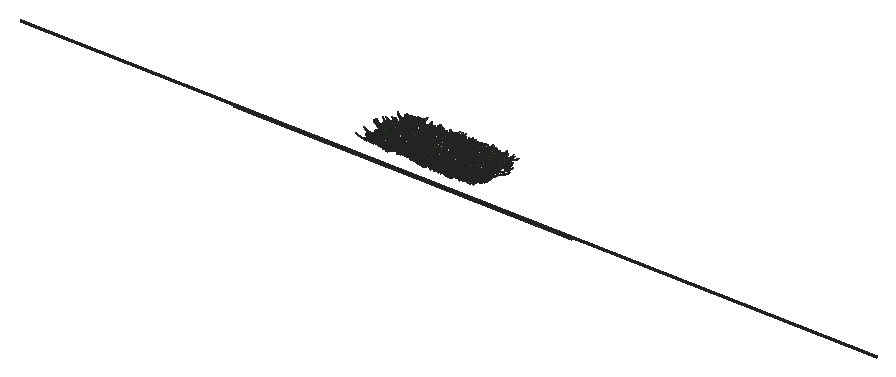
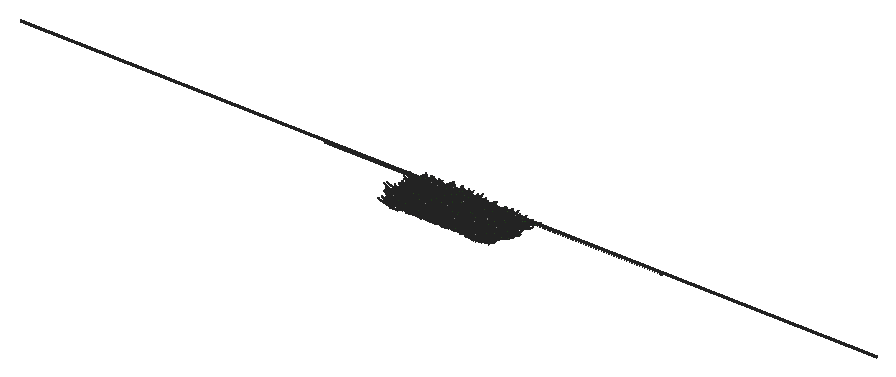
# SketchUp Ruby script. Lengths in inches.
U = 1.inch
M = Sketchup.active_model
def pt(a) = Geom::Point3d.new(a.map { |v| v * U })
def face(e, loops, mat)
  f = e.add_face(loops[0].map { |a| pt(a) })
  loops[1..].each { |l| e.add_face(l.map { |a| pt(a) }).erase! }
  f.material = f.back_material = mat if mat
  f
end
# faces: each face lists its corners as indices into pts; further lists are holes
def faces(e, pts, list, mat = nil) = list.each { |f| face(e, (f[0].is_a?(Array) ? f : [f]).map { |l| l.map { |i| pts[i] } }, mat) }
# xy, xz, yz: faces in a plane at the given z, y or x. An outline is a flat list of corners, or four numbers for a rectangle; further outlines are holes
def ring(l) = l.size == 4 ? [[l[0], l[1]], [l[2], l[1]], [l[2], l[3]], [l[0], l[3]]] : l.each_slice(2).to_a
def flat(e, list, mat, &to3) = list.each { |f| face(e, (f[0].is_a?(Array) ? f : [f]).map { |l| ring(l).map { |u, v| to3.(u, v) } }, mat) }
def xy(e, z, list, mat = nil) = flat(e, list, mat) { |x, y| [x, y, z] }
def xz(e, y, list, mat = nil) = flat(e, list, mat) { |x, z| [x, y, z] }
def yz(e, x, list, mat = nil) = flat(e, list, mat) { |y, z| [x, y, z] }
def lines(e, pts, list) = list.each { |a, b| e.add_line(pt(pts[a]), pt(pts[b])) }
# prism: a flat outline (further loops are holes) pulled along v
def prism(e, loops, v, mat = nil)
  f = face(e, loops, mat); d = Geom::Vector3d.new(v.map { |x| x * U })
  f.pushpull(f.normal.samedirection?(d) ? d.length : -d.length)
end
def box(e, o, s, mat = nil) = prism(e, [[o, [o[0] + s[0], o[1], o[2]], [o[0] + s[0], o[1] + s[1], o[2]], [o[0], o[1] + s[1], o[2]]]], [0, 0, s[2]], mat)
def at(x, y, z, deg = 0) = Geom::Transformation.translation(pt([x, y, z])) * Geom::Transformation.rotation(ORIGIN, Z_AXIS, deg.degrees)
def axes(o, x, y, z) = Geom::Transformation.new([*x, 0, *y, 0, *z, 0, *pt(o).to_a, 1])
def part(name) = M.definitions.add(name)
# library, detail: a bought-in or finely detailed component or shape, given as its bounding box
def library(name, o, s) = part(name).tap { |d| box(d.entities, o, s) }
def detail(e, o, s) = box(e.add_group.entities, o, s)
def put(e, d, t, mat = nil) = e.add_instance(d, t).tap { |i| i.material = mat if mat }
def group(e, t, mat = nil) = e.add_group.tap { |g| g.transformation = t; g.material = mat if mat }.entities
root = M.entities
M.materials.add("Material82").color = [68, 110, 58]
M.materials.add("Material83").color = [48, 90, 38]
M.materials.add("Material84").color = [68, 110, 48]
M.materials.add("Material85").color = [48, 90, 48]
M.materials.add("Material86").color = [58, 110, 58]
M.materials.add("Material87").color = [58, 90, 38]
M.materials.add("Material88").color = [68, 100, 58]
M.materials.add("Material89").color = [48, 100, 38]
c1 = part("grass00")
p = [[-0.6875,0.15,0],[-0.56,0.08,5.52],[-0.04,0.03,2.76],[0.48,-0.02,0],[0.35,-0.02,5.52],[-0.1,-0.14,5.52],
  [-0.12,0.65,8.37],[-0.42,0.65,8.37]]
faces(c1.entities,p,[[0,1,2,3],[3,2,4],[1,5,2],[5,4,2],[1,6,5],[4,5,6],[7,6,1]])
c2 = part("Group16\#1")
put(c2.entities,c1,axes([1.44,-0.61,-0.01],[0.05352,0.12609,0],[-0.10704,0.04543,0.07239],[0.06664,-0.02828,0.11628]),"Material85")
put(c2.entities,c1,axes([0.76,-0.15,-0.01],[0.04676,0.24062,0],[-0.23162,0.04501,0.06642],[0.0652,-0.01267,0.23595]),"Material82")
put(c2.entities,c1,axes([0.79,0.01,-0.01],[-0.00606,0.34651,0],[-0.34381,-0.00602,0.0432],[0.04319,0.00076,0.34386]))
put(c2.entities,c1,axes([1,0.23,-0.01],[-0.07192,0.31144,0],[-0.28722,-0.06632,0.1236],[0.12043,0.02781,0.29478]),"Material84")
put(c2.entities,c1,axes([1.66,0.77,-0.01],[-0.13828,0.29651,0],[-0.21551,-0.1005,0.22471],[0.20365,0.09498,0.23779]),"Material89")
put(c2.entities,c1,axes([0.6875,0.52,-0.01],[-0.18126,0.24051,0],[-0.22746,-0.17142,0.09788],[0.07817,0.05891,0.28481]),"Material84")
put(c2.entities,c1,axes([0.68,0.78,-0.01],[-0.215,0.18688,0],[-0.12385,-0.14248,0.21334],[0.13995,0.16101,0.18878]),"Material82")
put(c2.entities,c1,axes([0.56,1,-0.01],[-0.13756,0.07624,0],[-0.06159,-0.11112,0.0927],[0.04494,0.08108,0.12705]),"Material84")
put(c2.entities,c1,axes([0.2,0.64,-0.01],[-0.23729,0.07254,0],[-0.05711,-0.18681,0.153],[0.04473,0.14632,0.19535]),"Material89")
put(c2.entities,c1,axes([0.0625,0.72,-0.01],[-0.28874,0.02525,0],[-0.02179,-0.24916,0.14647],[0.01276,0.14591,0.25012]),"Material82")
put(c2.entities,c1,axes([-0.08,0.62,-0.01],[-0.34089,-0.04187,0],[0.03255,-0.26504,0.216],[-0.02633,0.21439,0.26703]),"Material89")
put(c2.entities,c1,axes([-0.34,0.98,-0.01],[-0.14314,-0.0493,0],[0.04397,-0.12769,0.06843],[-0.02228,0.0647,0.13505]),"Material89")
put(c2.entities,c1,axes([-0.87,1.45,-0.01],[-0.23488,-0.14114,0],[0.13761,-0.22901,0.06087],[-0.03135,0.05217,0.26717]))
put(c2.entities,c1,axes([-0.72,0.77,-0.01],[-0.14208,-0.13251,0],[0.07209,-0.0773,0.16301],[-0.11118,0.11922,0.1057]),"Material89")
put(c2.entities,c1,axes([-0.62,0.43,-0.01],[-0.14845,-0.21203,0],[0.18654,-0.13061,0.12304],[-0.10079,0.07057,0.22772]),"Material82")
put(c2.entities,c1,axes([-0.68,0.29,-0.01],[-0.13639,-0.32136,0],[0.31723,-0.13464,0.05579],[-0.05136,0.0218,0.34462]),"Material83")
put(c2.entities,c1,axes([-0.64,0.125,-0.01],[-0.0458,-0.23569,0],[0.22124,-0.043,0.08276],[-0.08124,0.01579,0.22538]),"Material86")
put(c2.entities,c1,axes([-1.6,-0.03,-0.01],[0.00576,-0.32897,0],[0.27526,0.00482,0.18018],[-0.18015,-0.00315,0.2753]),"Material84")
put(c2.entities,c1,axes([-1.36,-0.31,-0.01],[0.05718,-0.24765,0],[0.18172,0.04196,0.17267],[-0.16825,-0.03885,0.1865]),"Material89")
put(c2.entities,c1,axes([-1.54,-0.72,-0.01],[0.06537,-0.14017,0],[0.13555,0.06321,0.03939],[-0.0357,-0.01665,0.14956]))
put(c2.entities,c1,axes([-1.19,-0.9,-0.01],[0.09597,-0.12735,0],[0.11214,0.08451,0.07557],[-0.06035,-0.04548,0.14042]),"Material88")
put(c2.entities,c1,axes([-0.47,-0.54,-0.01],[0.11588,-0.10072,0],[0.0618,0.0711,0.12124],[-0.07953,-0.0915,0.0942]))
put(c2.entities,c1,axes([-0.47,-0.84,-0.01],[0.11927,-0.0661,0],[0.06603,0.11913,0.00646],[-0.00313,-0.00565,0.13621]),"Material84")
put(c2.entities,c1,axes([-0.38,-1.24,-0.01],[0.28037,-0.08571,0],[0.0618,0.20215,0.20315],[-0.05939,-0.19428,0.21139]),"Material88")
put(c2.entities,c1,axes([-0.06,-0.66,-0.01],[0.22719,-0.01987,0],[0.01247,0.14255,0.17758],[-0.01547,-0.17691,0.1431]),"Material87")
put(c2.entities,c1,axes([0.11,-0.89,-0.01],[0.14882,0.01828,0],[-0.01058,0.08611,0.12229],[0.01491,-0.12138,0.08676]),"Material85")
put(c2.entities,c1,axes([0.25,-0.72,-0.01],[0.20481,0.07053,0],[-0.06206,0.18022,0.10291],[0.03351,-0.0973,0.1906]),"Material85")
put(c2.entities,c1,axes([0.85,-1.42,-0.01],[0.16481,0.09904,0],[-0.09472,0.15762,0.05616],[0.02893,-0.04814,0.18389]),"Material84")
put(c2.entities,c1,axes([1.01,-1.09,-0.01],[0.21858,0.20385,0],[-0.17495,0.1876,0.15339],[0.10462,-0.11218,0.25652]),"Material89")
put(c2.entities,c1,axes([1.01,-0.71,-0.01],[0.08733,0.12473,0],[-0.06445,0.04512,0.13037],[0.1068,-0.07477,0.07867]),"Material85")
c3 = part("Group15\#1")
put(c3.entities,c2,at(0,0,0))
c4 = part("3darcstudiotree_grass00\#1")
put(c4.entities,c3,at(0,0,0))
xz(root,273.41,[[626.68,-39.125,848.97,-38.61],[486.41,-38.1875,1048.66,-37.86],[486.41,-37.86,1048.66,-37.24]])
put(root,c4,axes([755.25,281.3125,-34.17],[3.22982,-1.36398,0],[2.52221,0.92889,-0.01281],[0.05669,0.02088,1.56626]))
put(root,c4,axes([763.375,281.07,-34.17],[0.45304,1.69594,0],[-3.37186,0.14009,-0.01763],[-0.11097,0.00461,1.60818]))
put(root,c4,axes([752.73,281.26,-34.17],[-2.98133,1.10226,0],[-2.6348,-1.10837,-0.04557],[-0.21161,-0.08902,1.96028]))
put(root,c4,axes([745.06,281.49,-34.17],[0.75696,1.65896,0],[-4.64105,0.32936,-0.03105],[-0.12997,0.00922,1.50318]))
put(root,c4,axes([773.35,281.36,-34.17],[-1.86859,1.14232,0],[-3.14905,-0.80116,-0.00439],[-0.02189,-0.00557,1.66469]))
put(root,c4,axes([719.16,282.96,-34.17],[3.31562,-0.63662,0],[1.81859,1.47309,-0.02466],[0.05194,0.04207,1.49812]))
put(root,c4,axes([769.54,282.6,-34.17],[2.60331,1.05125,0],[-2.58261,0.9947,-0.01838],[-0.08057,0.03103,1.65818]))
put(root,c4,axes([734.7,282.9375,-34.17],[4.09444,0.12503,0],[-0.31641,1.61154,-0.0417],[-0.02006,0.10219,1.91485]))
put(root,c4,axes([755.98,283.15,-34.17],[3.14565,-0.76847,0],[1.85222,1.17921,-0.00486],[0.01386,0.00882,1.42853]))
put(root,c4,axes([738.35,282.67,-34.17],[-0.14266,1.36173,0],[-4.10184,-0.06683,-0.00296],[-0.01424,-0.00023,1.47961]))
put(root,c4,axes([722.52,282.6,-34.17],[-3.65106,0.9561,0],[-2.55118,-1.5152,-0.05111],[-0.12576,-0.07469,1.53759]))
put(root,c4,axes([750.39,282.95,-34.17],[-3.45178,0.2701,0],[-0.90786,-1.80446,-0.05548],[-0.0508,-0.10098,1.6451]))
put(root,c4,axes([727.26,283.58,-34.17],[3.35024,-0.43777,0],[1.10858,1.31952,-0.03222],[0.06859,0.08164,1.78787]))
put(root,c4,axes([713.76,283.2,-34.17],[-4.08016,-0.15242,0],[0.34321,-1.42893,-0.02721],[0.0124,-0.05162,1.31849]))
put(root,c4,axes([772.58,283.29,-34.17],[-0.10583,1.54224,0],[-3.7996,-0.04055,-0.00627],[-0.03571,-0.00038,1.62459]))
put(root,c4,axes([743.97,283.65,-34.17],[-2.56709,-0.87628,0],[2.75862,-1.25691,-0.00422],[0.01164,-0.0053,1.33295]))
put(root,c4,axes([762.34,283.9,-34.17],[2.94971,1.39882,0],[-3.26889,1.07209,-0.02991],[-0.14108,0.04627,1.95467]))
put(root,c4,axes([739.51,284.71,-34.17],[3.68364,0.44666,0],[-1.28613,1.64968,-0.02064],[-0.02718,0.03487,1.46981]))
put(root,c4,axes([756.35,285.1,-34.17],[1.53079,-1.5017,0],[4.19952,0.6658,-0.01772],[0.08663,0.01374,1.7874]))
put(root,c4,axes([717.34,284.68,-34.17],[-0.8053,1.43922,0],[-4.1788,-0.36366,-0.05256],[-0.20936,-0.01822,1.30827]))
put(root,c4,axes([752.53,285.36,-34.17],[1.13972,-1.41461,0],[4.50389,0.56436,-0.03698],[0.18209,0.02282,1.82987]))
put(root,c4,axes([734.63,285.26,-34.17],[3.61655,0.77067,0],[-2.16585,1.58076,-0.05913],[-0.11484,0.08382,1.39517]))
put(root,c4,axes([745.85,285.29,-34.17],[-1.56362,-1.21345,0],[3.6466,-0.73082,-0.00876],[0.03709,-0.00743,1.45672]))
put(root,c4,axes([774.84,285.4,-34.17],[-3.61232,0.8121,0],[-2.24589,-1.55373,-0.01918],[-0.05035,-0.03483,1.80194]))
put(root,c4,axes([766.03,286.01,-34.17],[3.57437,0.42668,0],[-1.04232,1.35805,-0.0422],[-0.08519,0.111,1.87907]))
put(root,c4,axes([727.7,286.11,-34.17],[2.52987,0.96809,0],[-2.35442,0.95693,-0.00683],[-0.03278,0.01332,1.74693]))
put(root,c4,axes([724.6875,285.88,-34.17],[0.40934,1.39565,0],[-3.638,0.16595,-0.04522],[-0.26335,0.01201,1.60941]))
put(root,c4,axes([764.01,285.87,-34.17],[-3.36311,0.85521,0],[-1.93534,-1.1837,-0.01497],[-0.0443,-0.0271,1.4615]))
put(root,c4,axes([713.21,286.76,-34.17],[0.83554,-1.66698,0],[4.46376,0.34798,-0.04547],[0.22573,0.0176,1.72572]))
put(root,c4,axes([768.86,286.72,-34.17],[-0.65586,-1.46962,0],[4.60144,-0.31938,-0.05842],[0.32577,-0.02261,1.98292]))
put(root,c4,axes([727.76,286.96,-34.17],[0.10079,1.33733,0],[-4.05045,0.04748,-0.05613],[-0.28184,0.0033,1.5259]))
put(root,c4,axes([773.53,287.11,-34.17],[-0.80891,1.58211,0],[-4.50454,-0.3582,-0.03197],[-0.1625,-0.01292,1.78572]))
put(root,c4,axes([762.92,287.18,-34.17],[-2.18902,1.07825,0],[-2.9207,-0.92221,-0.02462],[-0.13408,-0.04234,1.95656]))
put(root,c4,axes([721.68,287.61,-34.17],[-2.79747,-0.82267,0],[2.4,-1.26929,-0.00029],[0.00098,-0.00052,1.69542]))
put(root,c4,axes([746.86,287.51,-34.17],[0.20899,1.64265,0],[-4.27343,0.08456,-0.03261],[-0.1888,0.00374,1.85888]))
put(root,c4,axes([735.6875,287.79,-34.17],[-3.83423,-0.51133,0],[1.38691,-1.61748,-0.06149],[0.1095,-0.1277,1.80385]))
put(root,c4,axes([758.12,288.25,-34.17],[0.38628,-1.42854,0],[3.50239,0.14729,-0.04937],[0.32013,0.01346,1.72169]))
put(root,c4,axes([718.66,287.69,-34.17],[-1.21632,1.56365,0],[-3.36368,-0.40694,-0.03727],[-0.21338,-0.02582,1.57911]))
put(root,c4,axes([741.22,287.77,-34.17],[-2.10873,0.99525,0],[-2.92476,-0.96381,-0.03387],[-0.14037,-0.04626,1.54303]))
put(root,c4,axes([733.14,289.03,-34.17],[4.32757,-0.42653,0],[1.12297,1.77206,-0.03338],[0.0321,0.05066,1.37691]))
put(root,c4,axes([753,288.3,-34.17],[-3.3677,0.38425,0],[-1.22656,-1.67195,-0.00573],[-0.0077,-0.0105,1.59925]))
put(root,c4,axes([750.55,289.42,-34.17],[4.24203,-0.02956,0],[0.08072,1.80172,-0.02875],[0.00231,0.05162,1.55972]))
put(root,c4,axes([730.76,289.23,-34.17],[-2.64283,-1.13535,0],[3.48014,-1.25993,-0.02326],[0.08818,-0.03192,1.82249]))
put(root,c4,axes([768.4,289.62,-34.17],[1.16933,-1.48396,0],[3.883,0.47588,-0.02169],[0.1048,0.01284,1.54236]))
put(root,c4,axes([755.74,289.61,-34.17],[3.86384,0.07818,0],[-0.23972,1.84255,-0.05168],[-0.01275,0.09801,1.68853]))
put(root,c4,axes([741.0625,289.94,-34.17],[3.33633,-0.58263,0],[1.85643,1.65335,-0.04981],[0.10311,0.09183,1.75709]))
put(root,c4,axes([718.1875,290.5,-34.17],[2.313,-1.43442,0],[2.99954,0.75225,-0.04064],[0.1888,0.04735,1.46692]))
put(root,c4,axes([773.14,290.52,-34.17],[0.21445,-1.64927,0],[3.6182,0.07317,-0.01161],[0.06174,0.00125,1.44612]))
put(root,c4,axes([744.34,290.38,-34.17],[2.09092,1.38555,0],[-3.43654,0.80658,-0.00188],[-0.01015,0.00238,1.87843]))
put(root,c4,axes([763.36,290.52,-34.17],[-2.42754,-1.16571,0],[2.71881,-0.88058,-0.021],[0.08634,-0.02796,1.40308]))
put(root,c4,axes([725.09,290.24,-34.17],[-2.97215,1.15542,0],[-3.15373,-1.26173,-0.01243],[-0.04576,-0.01831,1.76595]))
put(root,c4,axes([764.41,291.39,-34.17],[3.8213,1.10557,0],[-2.37941,1.27911,-0.00415],[-0.01079,0.0058,1.32509]))
put(root,c4,axes([717.7,291.5,-34.17],[3.43029,0.99275,0],[-1.97308,1.06035,-0.01519],[-0.04853,0.02608,1.34969]))
put(root,c4,axes([772.67,291.5,-34.17],[-3.1974,-0.52057,0],[1.31873,-1.25975,-0.01181],[0.03016,-0.02882,1.73426]))
put(root,c4,axes([751.76,291.51,-34.17],[-3.96689,-0.26306,0],[0.64548,-1.51387,-0.0114],[0.01279,-0.03,1.97478]))
put(root,c4,axes([744.57,292.32,-34.17],[3.4734,-0.75241,0],[2.06047,1.47936,-0.02691],[0.07219,0.05183,1.78778]))
put(root,c4,axes([730.22,292.4375,-34.17],[1.26532,-1.44178,0],[3.12553,0.42661,-0.00044],[0.00223,0.0003,1.32507]))
put(root,c4,axes([721.66,292.03,-34.17],[2.61816,1.29298,0],[-2.60516,0.82044,-0.01421],[-0.06264,0.01973,1.40932]))
put(root,c4,axes([738.7,292.6,-34.17],[2.17735,-1.14497,0],[3.55677,1.05197,-0.03529],[0.11494,0.03399,1.35654]))
put(root,c4,axes([736.05,291.86,-34.17],[-3.45507,0.18922,0],[-0.60525,-1.7188,-0.02154],[-0.01288,-0.03658,1.4342]))
put(root,c4,axes([758.55,291.99,-34.17],[0.41177,1.61489,0],[-3.5087,0.13914,-0.04963],[-0.27633,0.01096,1.47912]))
put(root,c4,axes([768.19,292.23,-34.17],[-3.24054,-0.28468,0],[0.77392,-1.37016,-0.02543],[0.03342,-0.05916,1.61262]))
put(root,c4,axes([729.84,293.65,-34.17],[3.40614,0.32781,0],[-0.81542,1.31776,-0.01459],[-0.02356,0.03807,1.75568]))
put(root,c4,axes([774.73,293.92,-34.17],[4.64374,0.18316,0],[-0.43015,1.69615,-0.02551],[-0.01161,0.04577,1.48132]))
put(root,c4,axes([741.5,293.4,-34.17],[-3.50392,-0.27669,0],[0.88512,-1.7433,-0.02406],[0.02146,-0.04227,1.53532]))
put(root,c4,axes([735.4375,293.52,-34.17],[1.33968,1.52005,0],[-3.16755,0.43419,-0.01128],[-0.07711,0.01057,1.81963]))
put(root,c4,axes([766.4,294.16,-34.17],[1.53865,-1.45346,0],[4.25105,0.69992,-0.03949],[0.18935,0.03118,1.7941]))
put(root,c4,axes([721.62,294,-34.17],[-3.43052,-0.93956,0],[2.00829,-1.14045,-0.00375],[0.01479,-0.0084,1.82358]))
put(root,c4,axes([749.93,294.53,-34.17],[-0.8562,-1.46222,0],[3.2715,-0.29793,-0.0292],[0.1741,-0.01586,1.53984]))
put(root,c4,axes([756.88,294.38,-34.17],[-3.12873,-1.31633,0],[2.88309,-1.0658,-0.03051],[0.12402,-0.04585,1.65027]))
put(root,c4,axes([716.5,294.17,-34.17],[1.08587,1.67228,0],[-4.264,0.43062,-0.00469],[-0.02209,0.00223,1.60422]))
put(root,c4,axes([713.79,294.57,-34.17],[-2.42435,1.35441,0],[-3.23148,-0.89962,-0.04566],[-0.20763,-0.0578,1.65042]))
put(root,c4,axes([746.87,294.8,-34.17],[-2.97303,0.61552,0],[-2.04085,-1.53313,-0.02543],[-0.06857,-0.05151,1.9093]))
put(root,c4,axes([729.625,295.45,-34.17],[0.04452,-1.40138,0],[3.5701,0.01764,-0.00992],[0.04898,0.00024,1.32167]))
put(root,c4,axes([763.46,294.86,-34.17],[-4.30499,0.20084,0],[-0.50439,-1.68151,-0.02284],[-0.01208,-0.04026,1.44864]))
put(root,c4,axes([753.09,295.68,-34.17],[-2.49551,-1.26471,0],[2.8619,-0.87828,-0.01663],[0.09126,-0.02801,1.89037]))
put(root,c4,axes([733.8125,296,-34.17],[3.17214,0.39156,0],[-1.05658,1.33127,-0.01935],[-0.04192,0.05282,1.92273]))
put(root,c4,axes([712.15,296.01,-34.17],[3.52761,0.55067,0],[-1.26989,1.26523,-0.04887],[-0.1287,0.12823,1.85053]))
put(root,c4,axes([720.16,296.8,-34.17],[3.22727,-0.96219,0],[2.40393,1.25403,-0.04167],[0.15655,0.08166,1.86151]))
put(root,c4,axes([765.95,296.79,-34.17],[1.36885,-1.43158,0],[3.98655,0.59286,-0.04892],[0.27754,0.04127,1.93615]))
put(root,c4,axes([761.17,296.19,-34.17],[-3.9685,0.8355,0],[-2.02289,-1.49439,-0.03463],[-0.09424,-0.06962,1.86049]))
put(root,c4,axes([725.1875,296.36,-34.17],[1.39622,1.62786,0],[-3.6301,0.48424,-0.04556],[-0.23124,0.03085,1.53888]))
put(root,c4,axes([739.57,296.34,-34.17],[-4.01589,0.275,0],[-0.74615,-1.69466,-0.05401],[-0.03733,-0.08478,1.3206]))
put(root,c4,axes([773.73,296.38,-34.17],[-3.10318,1.24143,0],[-2.60712,-1.01358,-0.05097],[-0.2393,-0.09303,1.80901]))
put(root,c4,axes([755.57,296.39,-34.17],[0.17144,1.84869,0],[-4.60552,0.06643,-0.0182],[-0.07619,0.0011,1.44668]))
put(root,c4,axes([746.52,296.81,-34.17],[2.02269,1.40625,0],[-2.88305,0.64496,-0.03898],[-0.27125,0.06068,1.98748]))
put(root,c4,axes([717.3,297.63,-34.17],[0.48715,-1.38403,0],[3.63737,0.19912,-0.0013],[0.00869,0.00048,1.85519]))
put(root,c4,axes([774.21,297.67,-34.17],[4.4529,0.04613,0],[-0.09862,1.48061,-0.04419],[-0.00818,0.12282,1.98467]))
put(root,c4,axes([763.3,297.87,-34.17],[-1.73285,-1.40976,0],[3.20349,-0.61242,-0.03263],[0.20579,-0.03934,1.87]))
put(root,c4,axes([741.37,297.76,-34.17],[0.25957,1.50579,0],[-3.94932,0.10588,-0.02807],[-0.1244,0.00334,1.3177]))
put(root,c4,axes([729.98,298.47,-34.17],[3.60093,0.62069,0],[-1.54425,1.39338,-0.01451],[-0.03218,0.02903,1.59989]))
put(root,c4,axes([769.54,298.41,-34.17],[-3.57377,-0.68668,0],[1.88387,-1.52489,-0.02869],[0.074,-0.0599,1.89824]))
put(root,c4,axes([722.57,298.84,-34.17],[4.25337,0.6683,0],[-1.56461,1.54873,-0.01606],[-0.02903,0.02874,1.54782]))
put(root,c4,axes([743.87,298.39,-34.17],[-2.10864,1.34219,0],[-3.56504,-0.87109,-0.01218],[-0.05259,-0.01285,1.59607]))
put(root,c4,axes([732.89,298.36,-34.17],[-2.73949,1.39402,0],[-3.69271,-1.12865,-0.03455],[-0.12332,-0.03769,1.58129]))
put(root,c4,axes([714.03,298.57,-34.17],[-4.29343,-0.7683,0],[1.85419,-1.61153,-0.00153],[0.00342,-0.00297,1.82565]))
put(root,c4,axes([750.54,299.13,-34.17],[-0.26486,1.49696,0],[-3.89065,-0.10706,-0.02357],[-0.1242,-0.00342,1.54387]))
put(root,c4,axes([718.5,299.89,-34.17],[2.27709,-1.12887,0],[2.96357,0.92974,-0.01848],[0.07518,0.02359,1.47553]))
put(root,c4,axes([757.24,299.24,-34.17],[-3.19374,0.7238,0],[-2.32014,-1.59223,-0.04948],[-0.1132,-0.07768,1.60238]))
put(root,c4,axes([755.24,300.34,-34.17],[4.72899,0.01401,0],[-0.03317,1.74196,-0.012],[-0.00046,0.02441,1.70791]))
put(root,c4,axes([733.2,300.48,-34.17],[-2.29669,-1.11112,0],[2.95834,-0.95105,-0.00371],[0.01505,-0.00484,1.4993]))
put(root,c4,axes([746.09,300.5,-34.17],[-3.17921,-1.35137,0],[3.1644,-1.15784,-0.01209],[0.04457,-0.01631,1.62724]))
put(root,c4,axes([772.52,300.76,-34.17],[-0.51556,-1.46046,0],[3.95081,-0.21691,-0.04493],[0.28513,-0.01565,1.91565]))
put(root,c4,axes([768.24,300.875,-34.17],[-1.16799,-1.2811,0],[3.57696,-0.50721,-0.0171],[0.1013,-0.01436,1.79343]))
put(root,c4,axes([763.83,300.54,-34.17],[0.87217,1.79185,0],[-4.36686,0.33058,-0.02457],[-0.1156,0.00875,1.59681]))
put(root,c4,axes([714.07,301.35,-34.17],[0.26653,-1.73376,0],[4.03869,0.09656,-0.02606],[0.1443,0.00345,1.68211]))
put(root,c4,axes([750.1875,301.02,-34.17],[-4.0045,-0.70324,0],[1.53901,-1.36302,-0.04343],[0.08424,-0.0746,1.35201]))
put(root,c4,axes([731.07,301.04,-34.17],[-0.93158,1.57452,0],[-3.64716,-0.33561,-0.02125],[-0.09909,-0.00912,1.34411]))
put(root,c4,axes([739.02,301.15,-34.17],[-1.92395,1.11114,0],[-2.73961,-0.73778,-0.01899],[-0.11099,-0.02989,1.75992]))
put(root,c4,axes([725.69,302.05,-34.17],[4.28281,-0.63976,0],[1.42181,1.48036,-0.01068],[0.01649,0.01717,1.31138]))
put(root,c4,axes([721.77,301.36,-34.17],[-3.74102,0.70585,0],[-1.92999,-1.5909,-0.05113],[-0.08819,-0.0727,1.33965]))
put(root,c4,axes([768.04,302.07,-34.17],[4.39904,-0.03006,0],[0.06093,1.38656,-0.04649],[0.00481,0.10943,1.57333]))
put(root,c4,axes([749.66,302.36,-34.17],[2.12424,-1.58648,0],[2.98317,0.62124,-0.03491],[0.20173,0.04201,1.65255]))
put(root,c4,axes([741.92,302.7,-34.17],[2.84805,-1.35819,0],[2.78081,0.90692,-0.04304],[0.21584,0.07039,1.76026]))
put(root,c4,axes([745.42,302.4,-34.17],[-1.97289,1.32597,0],[-3.97358,-0.91953,-0.01374],[-0.05147,-0.01191,1.50009]))
put(root,c4,axes([730.74,302.52,-34.17],[-4.13794,-0.2249,0],[0.58111,-1.66288,-0.00876],[0.00496,-0.01418,1.32289]))
put(root,c4,axes([755.37,302.74,-34.17],[1.47307,1.52241,0],[-3.55442,0.5349,-0.03212],[-0.18221,0.02742,1.73128]))
put(root,c4,axes([716.82,302.92,-34.17],[-4.03021,-0.53258,0],[1.1352,-1.33605,-0.02118],[0.04192,-0.04934,1.66873]))
put(root,c4,axes([771.67,303.0625,-34.17],[-4.17671,-0.8199,0],[2.05439,-1.62767,-0.0574],[0.10467,-0.08292,1.41402]))
put(root,c4,axes([760.75,303.1,-34.17],[-1.70053,1.52985,0],[-3.13018,-0.54115,-0.01229],[-0.08699,-0.01504,1.9803]))
put(root,c4,axes([736,303.53,-34.17],[-0.83712,1.35251,0],[-3.5635,-0.34303,-0.03757],[-0.17469,-0.01682,1.3158]))
put(root,c4,axes([774.88,304.51,-34.17],[1.76506,-1.25364,0],[3.37171,0.73833,-0.03203],[0.17156,0.03757,1.771]))
put(root,c4,axes([718.03,304.68,-34.17],[4.01997,0.45296,0],[-1.05214,1.45226,-0.01128],[-0.01738,0.02399,1.61003]))
put(root,c4,axes([769.39,304.58,-34.17],[-3.73914,-0.79189,0],[1.71097,-1.25649,-0.0264],[0.09118,-0.06696,1.979]))
put(root,c4,axes([746.15,304.67,-34.17],[-2.5712,-1.27561,0],[3.33499,-1.0455,-0.01168],[0.0385,-0.01207,1.34439]))
put(root,c4,axes([725.11,305.08,-34.17],[-1.28823,-1.73919,0],[3.44626,-0.39701,-0.03009],[0.18497,-0.02131,1.72353]))
put(root,c4,axes([752.88,305.2,-34.17],[4.6709,-0.11713,0],[0.23839,1.47848,-0.03177],[0.01367,0.08477,1.90853]))
put(root,c4,axes([758.35,304.68,-34.17],[-1.61807,1.52118,0],[-3.6405,-0.60227,-0.04701],[-0.26943,-0.04457,1.83905]))
put(root,c4,axes([764.2,305.29,-34.17],[0.02605,-1.38879,0],[4.64619,0.01356,-0.04606],[0.23946,0.0007,1.81052]))
put(root,c4,axes([739.63,305.15,-34.17],[-4.087,-0.33484,0],[0.93219,-1.7696,-0.02537],[0.02744,-0.05209,1.82613]))
put(root,c4,axes([736.76,305.8,-34.17],[3.08356,-0.59749,0],[1.85245,1.48689,-0.05746],[0.15906,0.12767,1.97658]))
put(root,c4,axes([727.58,305.67,-34.17],[-1.97401,-1.44609,0],[3.51216,-0.74566,-0.02018],[0.11603,-0.02463,1.95264]))
put(root,c4,axes([772.93,306.49,-34.17],[3.31436,0.96989,0],[-2.30719,1.22623,-0.02502],[-0.09786,0.05201,1.90511]))
put(root,c4,axes([730.95,306.57,-34.17],[1.53583,1.49996,0],[-3.93703,0.62697,-0.05886],[-0.22971,0.03658,1.33951]))
put(root,c4,axes([752.15,306.44,-34.17],[-3.7951,0.9119,0],[-2.12877,-1.37789,-0.05764],[-0.17628,-0.1141,1.8024]))
put(root,c4,axes([738.61,306.49,-34.17],[-0.37072,1.84099,0],[-4.27519,-0.13389,-0.01448],[-0.06545,-0.00205,1.45727]))
put(root,c4,axes([762.625,307.01,-34.17],[3.34775,0.73741,0],[-1.81639,1.28251,-0.02091],[-0.0568,0.0401,1.55496]))
put(root,c4,axes([718.35,307.36,-34.17],[4.2861,-0.44175,0],[0.90749,1.36943,-0.02428],[0.0455,0.06867,1.99391]))
put(root,c4,axes([756.71,307.12,-34.17],[-1.61628,-1.19973,0],[3.67441,-0.7699,-0.00698],[0.03732,-0.00782,1.8873]))
put(root,c4,axes([732.95,306.72,-34.17],[-2.8718,1.45727,0],[-2.81901,-0.86401,-0.03149],[-0.12433,-0.03811,1.33797]))
put(root,c4,axes([723.12,307.03,-34.17],[-0.09975,1.34747,0],[-4.08432,-0.04703,-0.00454],[-0.02466,-0.00028,1.66362]))
put(root,c4,axes([746.71,307.62,-34.17],[1.08869,1.44245,0],[-3.40274,0.39943,-0.00785],[-0.05372,0.00631,1.89978]))
put(root,c4,axes([767.05,307.93,-34.17],[-2.53143,-1.15701,0],[3.22557,-1.09761,-0.03179],[0.10043,-0.03417,1.33245]))
put(root,c4,axes([728.47,308.66,-34.17],[3.01451,-0.88182,0],[2.30556,1.22582,-0.02804],[0.08966,0.04767,1.55696]))
put(root,c4,axes([766.45,308.59,-34.17],[4.54472,-0.07638,0],[0.17813,1.64846,-0.04096],[0.00957,0.08859,1.72127]))
put(root,c4,axes([740.9,308.76,-34.17],[-0.69027,-1.34957,0],[4.18043,-0.33255,-0.04603],[0.23408,-0.01862,1.65834]))
put(root,c4,axes([749.61,308.78,-34.17],[3.97101,0.68213,0],[-1.55734,1.41002,-0.04191],[-0.07595,0.06876,1.32656]))
put(root,c4,axes([736.06,308.65,-34.17],[-3.97452,0.57658,0],[-1.26948,-1.361,-0.04924],[-0.12234,-0.13116,1.98345]))
put(root,c4,axes([757.02,309.19,-34.17],[3.23921,0.6316,0],[-1.61427,1.28761,-0.03066],[-0.08714,0.06951,1.75054]))
put(root,c4,axes([746.2,309.04,-34.17],[-3.47552,-0.34069,0],[1.08655,-1.72393,-0.01735],[0.02109,-0.03347,1.70162]))
put(root,c4,axes([722.49,309.39,-34.17],[-2.1448,1.18286,0],[-3.37437,-0.95161,-0.05929],[-0.21963,-0.06194,1.41608]))
put(root,c4,axes([717.58,310.01,-34.17],[2.25028,1.20461,0],[-3.26486,0.94856,-0.0323],[-0.12798,0.03718,1.496]))
put(root,c4,axes([771.48,309.84,-34.17],[-2.56609,1.18757,0],[-3.37526,-1.13431,-0.01912],[-0.05922,-0.0199,1.35238]))
